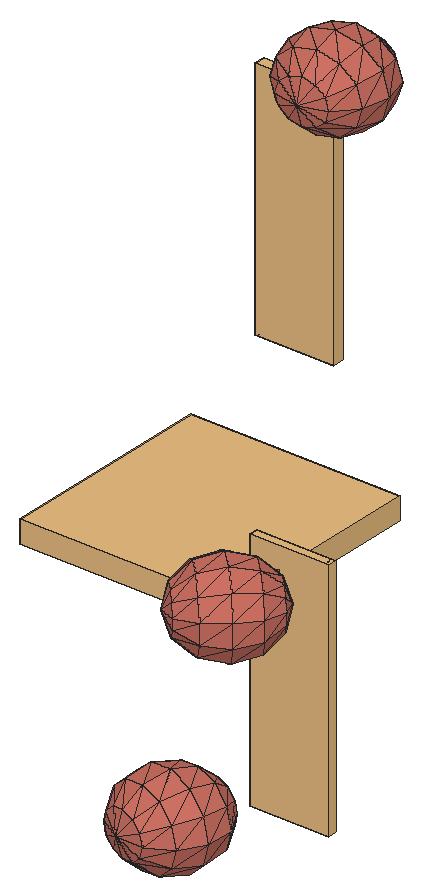
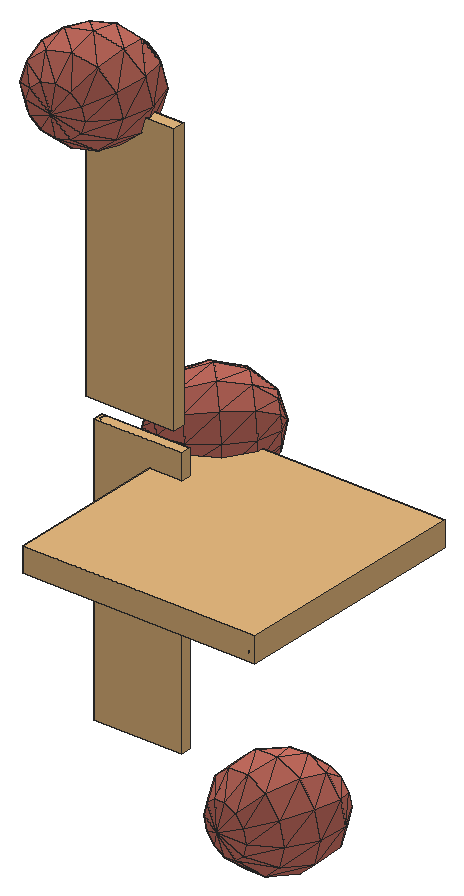
# SketchUp Ruby script. Lengths in inches.
U = 1.inch
M = Sketchup.active_model
def pt(a) = Geom::Point3d.new(a.map { |v| v * U })
def face(e, loops, mat)
  f = e.add_face(loops[0].map { |a| pt(a) })
  loops[1..].each { |l| e.add_face(l.map { |a| pt(a) }).erase! }
  f.material = f.back_material = mat if mat
  f
end
# faces: each face lists its corners as indices into pts; further lists are holes
def faces(e, pts, list, mat = nil) = list.each { |f| face(e, (f[0].is_a?(Array) ? f : [f]).map { |l| l.map { |i| pts[i] } }, mat) }
# xy, xz, yz: faces in a plane at the given z, y or x. An outline is a flat list of corners, or four numbers for a rectangle; further outlines are holes
def ring(l) = l.size == 4 ? [[l[0], l[1]], [l[2], l[1]], [l[2], l[3]], [l[0], l[3]]] : l.each_slice(2).to_a
def flat(e, list, mat, &to3) = list.each { |f| face(e, (f[0].is_a?(Array) ? f : [f]).map { |l| ring(l).map { |u, v| to3.(u, v) } }, mat) }
def xy(e, z, list, mat = nil) = flat(e, list, mat) { |x, y| [x, y, z] }
def xz(e, y, list, mat = nil) = flat(e, list, mat) { |x, z| [x, y, z] }
def yz(e, x, list, mat = nil) = flat(e, list, mat) { |y, z| [x, y, z] }
def lines(e, pts, list) = list.each { |a, b| e.add_line(pt(pts[a]), pt(pts[b])) }
# prism: a flat outline (further loops are holes) pulled along v
def prism(e, loops, v, mat = nil)
  f = face(e, loops, mat); d = Geom::Vector3d.new(v.map { |x| x * U })
  f.pushpull(f.normal.samedirection?(d) ? d.length : -d.length)
end
def box(e, o, s, mat = nil) = prism(e, [[o, [o[0] + s[0], o[1], o[2]], [o[0] + s[0], o[1] + s[1], o[2]], [o[0], o[1] + s[1], o[2]]]], [0, 0, s[2]], mat)
def at(x, y, z, deg = 0) = Geom::Transformation.translation(pt([x, y, z])) * Geom::Transformation.rotation(ORIGIN, Z_AXIS, deg.degrees)
def axes(o, x, y, z) = Geom::Transformation.new([*x, 0, *y, 0, *z, 0, *pt(o).to_a, 1])
def part(name) = M.definitions.add(name)
# library, detail: a bought-in or finely detailed component or shape, given as its bounding box
def library(name, o, s) = part(name).tap { |d| box(d.entities, o, s) }
def detail(e, o, s) = box(e.add_group.entities, o, s)
def put(e, d, t, mat = nil) = e.add_instance(d, t).tap { |i| i.material = mat if mat }
def group(e, t, mat = nil) = e.add_group.tap { |g| g.transformation = t; g.material = mat if mat }.entities
root = M.entities
M.materials.add("green").color = [174, 139, 102]
M.materials.add("vio").color = [206, 114, 100]
c1 = library("3DGeom~125_Defintion",[-500,-52.11,-487.65],[1000,104.22,975.3])
c2 = part("3DGeom~126_Defintion")
p = [[-471.41,-45.23,-481.51],[-492.01,-24.59,-479.28],[-477.71,-31.47,-487.65],[-471.41,-45.23,-481.51],[-477.71,-31.47,-487.65],[-472.84,-38.35,-486.35],
  [-492.01,-24.59,-479.28],[-484.73,-26.43,-485.0625],[-477.71,-31.47,-487.65],[-479.4,-52.11,-467],[-492.01,-24.59,-479.28],[-471.41,-45.23,-481.51],
  [-479.4,-52.11,-467],[-471.41,-45.23,-481.51],[-473.8125,-50.26,-474.43],[-493.7,-45.23,-458.63],[-492.01,-24.59,-479.28],[-479.4,-52.11,-467],
  [-500,-31.47,-464.77],[-492.01,-24.59,-479.28],[-493.7,-45.23,-458.63],[-492.01,-24.59,-479.28],[-497.6,-26.43,-471.85],[-493.7,-45.23,-458.63],
  [-479.4,-52.11,-467],[-486.68,-50.26,-461.22],[-493.7,-45.23,-458.63],[-498.57,-38.35,-459.93],[487.9375,29.11,475.22],[497.875,5.67,462.61],
  [500,13.48,461.23],[487.9375,29.11,475.22],[498.68,21.29,463.39],[487.9375,29.11,475.22],[492.87,-0.05,467.15],[497.875,5.67,462.61],
  [487.9375,29.11,475.22],[498.68,21.29,463.39],[494.26,27.01,468.51],[487.9375,29.11,475.22],[486.33,-2.15,473.66],[492.87,-0.05,467.15],
  [487.9375,29.11,475.22],[480,-0.05,480.37],[486.33,-2.15,473.66],[487.9375,29.11,475.22],[475.59,5.67,485.49],[480,-0.05,480.37],
  [487.9375,29.11,475.22],[474.26,13.48,487.65],[475.59,5.67,485.49],[487.9375,29.11,475.22],[476.39,21.29,486.27],[474.26,13.48,487.65],
  [487.9375,29.11,475.22],[481.39,27.01,481.72],[476.39,21.29,486.27]]
faces(c2.entities,p,[[0,1,2],[3,4,5],[6,7,8],[9,10,11],[12,13,14],[15,16,17],[18,19,20],[21,18,22],
  [23,24,25],[18,26,27],[28,29,30],[31,30,32],[33,34,35],[36,37,38],[39,40,41],[42,43,44],
  [45,46,47],[48,49,50],[51,52,53],[54,55,56]],"green")
c3 = part("3DGeom~196_Defintion")
p = [[141.97,-189.5,-442.47],[-141.24,0,-495.8],[125.58,0,-500],[368.22,-109.41,-337.01],[368.22,-109.41,-337.01],[358.76,0,-370.22],
  [-122.32,218.8125,-429.38],[141.97,189.5,-442.47],[358.76,0,-370.22],[-122.32,-218.81,-429.38],[-370.22,0,-358.76],[-353.83,189.5,-301.23],
  [186.74,-328.22,-285.3125],[394.07,-189.5,-246.27],[394.07,-189.5,-246.27],[368.22,-109.41,-337.01],[358.76,0,-370.22],[368.22,109.41,-337.01],
  [368.22,109.41,-337.01],[186.74,328.22,-285.3125],[-70.62,378.99,-247.9],[-70.62,378.99,-247.9],[186.74,328.22,-285.3125],[-70.62,-378.99,-247.9],
  [-353.83,-189.5,-301.23],[-309.0625,328.22,-144.07],[-309.0625,328.22,-144.07],[-70.62,378.99,-247.9],[368.22,-109.41,-337.01],[358.76,0,-370.22],
  [495.8,0,-141.24],[368.22,109.41,-337.01],[-353.83,-189.5,-301.23],[-500,0,-125.58],[-370.22,0,-358.76],[-370.22,0,-358.76],
  [-490.54,109.41,-92.37],[-370.22,0,-358.76],[-353.83,189.5,-301.23],[394.07,-189.5,-246.27],[394.07,189.5,-246.27],[368.22,109.41,-337.01],
  [186.74,328.22,-285.3125],[394.07,189.5,-246.27],[-309.0625,-328.22,-144.07],[-309.0625,-328.22,-144.07],[-490.54,-109.41,-92.37],[-353.83,-189.5,-301.23],
  [-353.83,-189.5,-301.23],[-353.83,189.5,-301.23],[-464.6875,189.5,-1.63],[-353.83,189.5,-301.23],[-309.0625,328.22,-144.07],[247.9,-378.99,-70.62],
  [-70.62,-378.99,-247.9],[186.74,-328.22,-285.3125],[429.38,-218.8125,-122.32],[247.9,-378.99,-70.62],[186.74,-328.22,-285.3125],[186.74,-328.22,-285.3125],
  [186.74,328.22,-285.3125],[247.9,378.99,-70.62],[186.74,328.22,-285.3125],[-70.62,378.99,-247.9],[0,437.625,0],[186.74,328.22,-285.3125],
  [247.9,378.99,-70.62],[0,-437.625,0],[-309.0625,-328.22,-144.07],[-70.62,-378.99,-247.9],[247.9,-378.99,-70.62],[-70.62,-378.99,-247.9],
  [-309.0625,328.22,-144.07],[-247.9,378.99,70.62],[429.38,218.8125,-122.32],[-247.9,-378.99,70.62],[-309.0625,-328.22,-144.07],[-247.9,-378.99,70.62],
  [-464.6875,-189.5,-1.63],[-309.0625,-328.22,-144.07],[-309.0625,-328.22,-144.07],[-309.0625,328.22,-144.07],[-429.38,218.8125,122.32],[-309.0625,328.22,-144.07],
  [-247.9,378.99,70.62],[464.6875,-189.5,1.63],[490.54,-109.41,92.37],[500,0,125.58],[464.6875,189.5,1.63],[490.54,109.41,92.37],
  [-495.8,0,141.24],[309.0625,328.22,144.07],[309.0625,-328.22,144.07],[247.9,-378.99,-70.62],[309.0625,-328.22,144.07],[247.9,378.99,-70.62],
  [70.62,378.99,247.9],[309.0625,328.22,144.07],[247.9,378.99,-70.62],[70.62,378.99,247.9],[-247.9,-378.99,70.62],[-429.38,-218.8125,122.32],
  [70.62,-378.99,247.9],[309.0625,-328.22,144.07],[-186.74,328.22,285.3125],[-186.74,328.22,285.3125],[70.62,378.99,247.9],[353.83,189.5,301.23],
  [-186.74,-328.22,285.3125],[-247.9,-378.99,70.62],[-186.74,-328.22,285.3125],[-247.9,378.99,70.62],[-394.07,189.5,246.27],[-247.9,378.99,70.62],
  [-394.07,189.5,246.27],[-186.74,328.22,285.3125],[353.83,-189.5,301.23],[370.22,0,358.76],[-186.74,-328.22,285.3125],[-394.07,-189.5,246.27],
  [-394.07,189.5,246.27],[-368.22,-109.41,337.01],[-368.22,-109.41,337.01],[-358.76,0,370.22],[-358.76,0,370.22],[-368.22,109.41,337.01],
  [-368.22,109.41,337.01],[-394.07,189.5,246.27],[353.83,-189.5,301.23],[70.62,-378.99,247.9],[309.0625,-328.22,144.07],[309.0625,328.22,144.07],
  [122.32,218.8125,429.38],[353.83,189.5,301.23],[309.0625,328.22,144.07],[70.62,378.99,247.9],[-141.97,-189.5,442.47],[-394.07,-189.5,246.27],
  [-186.74,-328.22,285.3125],[-368.22,-109.41,337.01],[-394.07,-189.5,246.27],[-186.74,328.22,285.3125],[-394.07,189.5,246.27],[-368.22,109.41,337.01],
  [122.32,-218.8125,429.38],[-186.74,-328.22,285.3125],[70.62,-378.99,247.9],[353.83,-189.5,301.23],[70.62,-378.99,247.9],[-141.97,189.5,442.47],
  [-186.74,-328.22,285.3125],[370.22,0,358.76],[353.83,-189.5,301.23],[353.83,189.5,301.23],[141.24,0,495.8],[353.83,189.5,301.23],
  [370.22,0,358.76],[-125.58,0,500],[-358.76,0,370.22],[370.22,0,358.76]]
faces(c3.entities,p,[[0,1,2],[3,0,2],[4,2,5],[2,1,6],[2,6,7],[8,2,7],[9,10,1],[0,9,1],
  [1,10,11],[1,11,6],[12,9,0],[13,12,0],[14,0,15],[16,7,17],[18,7,19],[7,6,20],
  [7,21,22],[23,24,9],[12,23,9],[9,24,10],[6,11,25],[6,26,27],[28,29,30],[29,31,30],
  [32,33,34],[35,33,36],[37,36,38],[39,28,30],[31,40,30],[41,42,43],[23,44,24],[45,46,47],
  [48,46,33],[49,36,50],[51,50,52],[53,54,55],[56,57,58],[56,59,39],[40,60,61],[62,63,64],
  [65,64,66],[67,68,69],[70,67,71],[63,72,73],[63,73,64],[56,39,30],[40,74,30],[40,61,74],
  [67,75,76],[77,78,79],[80,78,46],[81,50,82],[83,82,84],[85,56,30],[86,85,30],[87,86,30],
  [74,88,30],[88,89,30],[89,87,30],[33,46,90],[36,33,90],[85,57,56],[74,91,88],[74,61,91],
  [46,78,90],[50,36,90],[92,67,93],[85,94,57],[95,96,97],[98,64,99],[100,101,78],[78,101,90],
  [82,50,90],[102,75,67],[103,102,67],[64,73,104],[64,105,106],[86,94,85],[88,107,89],[88,91,107],
  [108,101,109],[102,110,75],[111,82,112],[113,114,115],[86,116,94],[87,116,86],[89,107,117],[89,117,87],
  [118,119,101],[101,119,90],[120,82,90],[87,117,116],[119,121,90],[122,123,90],[124,125,90],[126,127,90],
  [128,129,130],[131,132,133],[134,135,132],[136,137,138],[136,139,140],[141,142,143],[144,145,146],[147,144,148],
  [135,141,149],[135,149,132],[144,136,150],[141,143,149],[151,144,152],[153,132,154],[155,154,156],[157,139,136],
  [157,158,139],[149,143,158],[159,154,144],[149,158,157],[154,136,144],[132,149,157],[132,157,154],[154,157,136]],"vio")
c4 = library("3DGeom~119_Defintion",[-23.33,-500,-162.27],[46.66,1000,324.54])
c5 = part("3DGeom~120_Defintion")
p = [[-7.96,-495.57,-128.3],[7.3,-500,-151.51],[5.77,-494.09,-119.66],[-7.2,-498.52,-144.22],[7.3,-500,-151.51],[-7.96,-495.57,-128.3],
  [7.3,-500,-151.51],[-7.2,-498.52,-144.22],[-0.95,-499.6,-149.76],[5.77,-494.09,-119.66],[7.3,-500,-151.51],[20.27,-495.57,-126.94],
  [7.3,-500,-151.51],[15.35,-499.6,-148.98],[21.03,-498.52,-142.87],[20.27,-495.57,-126.94],[7.3,-500,-151.51],[21.03,-498.52,-142.87],
  [-7.2,-498.52,-144.22],[-7.96,-495.57,-128.3],[-9.76,-497.04,-136.37],[20.27,-495.57,-126.94],[21.03,-498.52,-142.87],[22.83,-497.04,-134.8],
  [-7.96,-495.57,-128.3],[5.77,-494.09,-119.66],[-2.28,-494.49,-122.18],[5.77,-494.09,-119.66],[20.27,-495.57,-126.94],[14.02,-494.49,-121.4],
  [-6.3,500,131.58],[-15.82,491.3,159.83],[-7.77,490.68,162.27],[-6.3,500,131.58],[-7.77,490.68,162.27],[0.48,491.3,160.61],
  [-6.3,500,131.58],[-21.52,493.01,153.92],[-15.82,491.3,159.83],[-6.3,500,131.58],[0.48,491.3,160.61],[6.71,493.01,155.28],
  [-6.3,500,131.58],[-23.33,495.34,146.14],[-21.52,493.01,153.92],[-6.3,500,131.58],[6.71,493.01,155.28],[9.26,495.34,147.71],
  [-6.3,500,131.58],[-20.78,497.67,138.57],[-23.33,495.34,146.14],[-6.3,500,131.58],[9.26,495.34,147.71],[7.45,497.67,139.93],
  [-6.3,500,131.58],[-14.55,499.375,133.24],[-20.78,497.67,138.57],[-6.3,500,131.58],[7.45,497.67,139.93],[1.75,499.375,134.03]]
faces(c5.entities,p,[[0,1,2],[3,4,5],[6,7,8],[9,10,11],[12,13,14],[15,16,17],[18,19,20],[21,22,23],
  [24,25,26],[27,28,29],[30,31,32],[33,34,35],[36,37,38],[39,40,41],[42,43,44],[45,46,47],
  [48,49,50],[51,52,53],[54,55,56],[57,58,59]],"green")
c6 = part("3DGeom~226_Defintion")
p = [[20.8,-212.46,-433.01],[-229.2,0,-445.02],[24.02,0,-500],[268.02,-184,-362.99],[268.02,-184,-362.99],[270.8,0,-421],
  [-231.98,184,-387.01],[20.8,212.47,-433.01],[270.8,0,-421],[-231.98,-184,-387.01],[-421,0,-270.8],[-422.61,106.23,-237.31],
  [-422.61,106.23,-237.31],[12.01,-368,-250],[260.4,-318.7,-204.5],[260.4,-318.7,-204.5],[268.02,-184,-362.99],[270.8,0,-421],
  [268.02,184,-362.99],[-239.6,318.7,-228.52],[268.02,184,-362.99],[12.01,368,-250],[-239.6,318.7,-228.52],[12.01,368,-250],
  [443.41,-106.23,-195.7],[268.02,-184,-362.99],[270.8,0,-421],[445.02,0,-229.2],[268.02,184,-362.99],[-239.6,-318.7,-228.52],
  [-239.6,-318.7,-228.52],[-422.61,-106.23,-237.31],[-231.98,-184,-387.01],[-422.61,-106.23,-237.31],[-231.98,184,-387.01],[-422.61,106.23,-237.31],
  [-427.01,184,-145.8],[-231.98,184,-387.01],[-239.6,318.7,-228.52],[439.02,-184,-104.2],[260.4,-318.7,-204.5],[443.41,106.23,-195.7],
  [260.4,318.7,-204.5],[268.02,184,-362.99],[12.01,368,-250],[260.4,318.7,-204.5],[-421,0,-270.8],[-422.61,-106.23,-237.31],
  [-500,0,-24.02],[-421,0,-270.8],[0,-424.93,0],[-239.6,-318.7,-228.52],[12.01,-368,-250],[250,-368,12.01],
  [12.01,-368,-250],[250,-368,12.01],[12.01,-368,-250],[260.4,-318.7,-204.5],[12.01,368,-250],[-239.6,318.7,-228.52],
  [-250,368,-12.01],[260.4,318.7,-204.5],[0,424.93,0],[-239.6,-318.7,-228.52],[-427.01,-184,-145.8],[-422.61,-106.23,-237.31],
  [-422.61,-106.23,-237.31],[500,0,24.02],[-250,-368,-12.01],[-239.6,-318.7,-228.52],[-250,-368,-12.01],[-239.6,-318.7,-228.52],
  [-239.6,318.7,-228.52],[-433.01,212.47,-20.8],[-239.6,318.7,-228.52],[-250,368,-12.01],[433.01,-212.47,20.8],[250,-368,12.01],
  [439.02,184,-104.2],[250,368,12.01],[260.4,318.7,-204.5],[250,368,12.01],[-250,-368,-12.01],[-433.01,-212.46,-20.8],
  [433.01,212.46,20.8],[-439.02,-184,104.2],[-443.41,-106.23,195.7],[-445.02,0,229.2],[-443.41,106.23,195.7],[-439.02,184,104.2],
  [-260.4,-318.7,204.5],[-250,-368,-12.01],[-260.4,-318.7,204.5],[-250,368,-12.01],[-12.01,-368,250],[-260.4,-318.7,204.5],
  [-250,368,-12.01],[-260.4,318.7,204.5],[-260.4,318.7,204.5],[239.6,-318.7,228.52],[239.6,-318.7,228.52],[250,-368,12.01],
  [-260.4,318.7,204.5],[-12.01,368,250],[250,368,12.01],[-12.01,368,250],[427.01,-184,145.8],[239.6,-318.7,228.52],
  [239.6,318.7,228.52],[250,368,12.01],[-12.01,368,250],[239.6,318.7,228.52],[427.01,184,145.8],[422.61,-106.23,237.31],
  [421,0,270.8],[422.61,106.23,237.31],[-268.01,-184,362.99],[-260.4,-318.7,204.5],[-268.01,-184,362.99],[-260.4,318.7,204.5],
  [231.99,184,387.01],[231.99,184,387.01],[-270.8,0,421],[-268.01,-184,362.99],[-270.8,0,421],[-268.01,184,362.99],
  [-260.4,318.7,204.5],[-268.01,184,362.99],[-20.8,-212.47,433.01],[-260.4,-318.7,204.5],[-12.01,-368,250],[-268.01,-184,362.99],
  [-260.4,-318.7,204.5],[-12.01,368,250],[-260.4,318.7,204.5],[-268.01,184,362.99],[231.99,-184,387.01],[-12.01,-368,250],
  [239.6,-318.7,228.52],[231.99,-184,387.01],[239.6,318.7,228.52],[-20.8,212.47,433.01],[231.99,184,387.01],[239.6,318.7,228.52],
  [-268.01,184,362.99],[-270.8,0,421],[421,0,270.8],[231.99,-184,387.01],[422.61,-106.23,237.31],[422.61,106.23,237.31],
  [229.2,0,445.02],[422.61,106.23,237.31],[421,0,270.8],[231.99,-184,387.01],[-12.01,-368,250],[421,0,270.8],
  [231.99,-184,387.01],[-24.02,0,500],[-270.8,0,421],[231.99,-184,387.01]]
faces(c6.entities,p,[[0,1,2],[3,0,2],[4,2,5],[2,1,6],[2,6,7],[8,2,7],[0,9,1],[9,10,1],
  [1,10,11],[1,12,6],[13,9,0],[14,13,0],[15,0,16],[17,7,18],[7,6,19],[20,7,21],
  [7,22,23],[24,25,26],[24,26,27],[27,26,28],[13,29,9],[30,31,32],[9,33,10],[34,35,36],
  [37,36,38],[39,40,25],[39,25,24],[27,28,41],[41,28,42],[43,44,45],[46,47,48],[35,49,48],
  [50,51,52],[53,50,54],[55,56,57],[58,59,60],[61,58,62],[58,60,62],[63,64,65],[66,64,48],
  [36,35,48],[24,27,67],[27,41,67],[50,68,69],[70,64,71],[72,36,73],[74,73,75],[76,77,40],
  [76,40,39],[41,42,78],[78,42,79],[80,62,81],[39,24,67],[41,78,67],[82,83,64],[64,83,48],
  [73,36,48],[76,39,67],[78,84,67],[78,79,84],[83,85,48],[85,86,48],[86,87,48],[87,88,48],
  [88,89,48],[89,73,48],[90,83,91],[92,85,83],[93,73,89],[94,68,50],[94,95,68],[96,89,97],
  [62,60,98],[99,94,50],[100,50,101],[62,102,103],[104,62,105],[106,107,77],[106,77,76],[84,79,108],
  [109,110,111],[106,76,67],[84,112,67],[84,108,112],[113,106,67],[114,113,67],[115,114,67],[112,115,67],
  [116,85,117],[118,86,85],[119,89,88],[113,107,106],[112,120,115],[112,108,121],[122,86,123],[124,87,86],
  [125,88,87],[126,88,127],[128,129,130],[128,131,132],[133,134,135],[136,137,138],[113,139,107],[140,141,142],
  [143,133,141],[144,87,145],[146,147,148],[149,142,150],[151,150,152],[153,128,154],[133,135,141],[155,150,156],
  [157,131,128],[157,158,131],[141,135,158],[150,128,159],[142,141,157],[142,157,150],[141,158,157],[150,157,128]],"vio")
c7 = part("3DGeom~229_Defintion")
p = [[135.68,-61.63,-498.07],[-132.16,91.58,-492.59],[133.7,52.87,-500],[363.74,0,-373.43],[180.3,153.22,-454.61],[-51.45,265.375,-413.98],
  [185.71,-159.63,-449.34],[-128.73,-106.76,-489.25],[-362.61,105.75,-353.2],[-269.41,306.43,-262.42],[-269.41,306.43,-262.42],[-42.08,-276.49,-404.84],
  [-358.65,-123.27,-349.34],[262.99,212.5,-374.0625],[91.78,368.07,-274.47],[91.78,368.07,-274.47],[270.39,-214.85,-366.86],[-51.45,265.375,-413.98],
  [-269.41,306.43,-262.42],[-104.02,425.01,-101.32],[-51.45,265.375,-413.98],[91.78,368.07,-274.47],[104.59,-372.13,-261.99],[-258.59,-319.26,-251.875],
  [-42.08,-276.49,-404.84],[104.59,-372.13,-261.99],[-258.59,-319.26,-251.875],[359.62,214.85,-279.94],[262.99,212.5,-374.0625],[259.15,372.13,-111.44],
  [262.99,212.5,-374.0625],[259.15,372.13,-111.44],[359.62,214.85,-279.94],[367.02,-212.5,-272.74],[449.71,-153.21,-192.19],[367.02,-212.5,-272.74],
  [363.74,0,-373.43],[496.3125,-52.87,-146.8],[363.74,0,-373.43],[494.33,61.64,-148.73],[363.74,0,-373.43],[359.62,214.85,-279.94],
  [444.3,159.63,-197.46],[363.74,0,-373.43],[363.74,0,-373.43],[367.02,-212.5,-272.74],[104.59,-372.13,-261.99],[270.39,-214.85,-366.86],
  [-358.65,-123.27,-349.34],[-495.9,91.58,-119.16],[-362.61,105.75,-353.2],[-362.61,105.75,-353.2],[-415.1875,265.38,-40.55],[-362.61,105.75,-353.2],
  [-415.1875,265.38,-40.55],[-269.41,306.43,-262.42],[-258.59,-319.26,-251.875],[-492.47,-106.76,-115.82],[-358.65,-123.27,-349.34],[-358.65,-123.27,-349.34],
  [405.8125,276.49,31.41],[259.15,372.13,-111.44],[89.24,429.7,86.92],[259.15,372.13,-111.44],[367.02,-212.5,-272.74],[271.96,-368.07,-98.97],
  [104.59,-372.13,-261.99],[271.96,-368.07,-98.97],[367.02,-212.5,-272.74],[-415.1875,265.38,-40.55],[-271.96,368.07,98.97],[104.59,-372.13,-261.99],
  [-89.24,-429.7,-86.92],[-258.59,-319.26,-251.875],[104.59,-372.13,-261.99],[-405.8125,-276.49,-31.41],[-258.59,-319.26,-251.875],[-258.59,-319.26,-251.875],
  [-405.8125,-276.49,-31.41],[492.47,106.75,115.82],[415.1875,-265.375,40.55],[271.96,-368.07,-98.97],[495.9,-91.58,119.16],[-496.3125,52.87,146.8],
  [-449.71,153.21,192.19],[-415.1875,265.38,-40.55],[-494.33,-61.64,148.73],[259.15,372.13,-111.44],[258.59,319.26,251.875],[405.8125,276.49,31.41],
  [259.15,372.13,-111.44],[258.59,319.26,251.875],[-104.59,372.13,261.99],[104.02,-425.01,101.32],[415.1875,-265.375,40.55],[-259.15,-372.13,111.44],
  [-405.8125,-276.49,-31.41],[-415.1875,265.38,-40.55],[-367.02,212.5,272.74],[-415.1875,265.38,-40.55],[-367.02,212.5,272.74],[-271.96,368.07,98.97],
  [-259.15,-372.13,111.44],[-444.3,-159.63,197.46],[358.65,123.27,349.34],[258.59,319.26,251.875],[415.1875,-265.375,40.55],[269.41,-306.43,262.42],
  [269.41,-306.43,262.42],[42.08,276.49,404.84],[42.08,276.49,404.84],[258.59,319.26,251.875],[-367.02,212.5,272.74],[-270.39,214.85,366.86],
  [-270.39,214.85,366.86],[-91.78,-368.07,274.47],[-259.15,-372.13,111.44],[-359.62,-214.85,279.94],[-359.62,-214.85,279.94],[362.61,-105.75,353.2],
  [269.41,-306.43,262.42],[-363.74,0,373.43],[-367.02,212.5,272.74],[258.59,319.26,251.875],[42.08,276.49,404.84],[128.73,106.76,489.25],
  [258.59,319.26,251.875],[358.65,123.27,349.34],[-104.59,372.13,261.99],[-270.39,214.85,366.86],[-185.71,159.63,449.34],[-104.59,372.13,261.99],
  [51.45,-265.375,413.98],[362.61,-105.75,353.2],[51.45,-265.375,413.98],[269.41,-306.43,262.42],[-367.02,212.5,272.74],[-363.74,0,373.43],
  [-262.99,-212.5,374.0625],[-359.62,-214.85,279.94],[51.45,-265.375,413.98],[-262.99,-212.5,374.0625],[-91.78,-368.07,274.47],[-359.62,-214.85,279.94],
  [-262.99,-212.5,374.0625],[-363.74,0,373.43],[358.65,123.27,349.34],[132.16,-91.58,492.59],[362.61,-105.75,353.2],[358.65,123.27,349.34],
  [362.61,-105.75,353.2],[51.45,-265.375,413.98],[-363.74,0,373.43],[-262.99,-212.5,374.0625],[-180.3,-153.22,454.61],[-363.74,0,373.43],
  [-133.7,-52.87,500],[-363.74,0,373.43],[-135.68,61.63,498.07],[-363.74,0,373.43],[-363.74,0,373.43],[51.45,-265.375,413.98],
  [-262.99,-212.5,374.0625],[51.45,-265.375,413.98]]
faces(c7.entities,p,[[0,1,2],[0,2,3],[2,4,3],[2,1,5],[2,5,4],[6,7,0],[6,0,3],[0,7,1],
  [7,8,1],[1,8,9],[1,10,5],[11,12,7],[6,11,7],[7,12,8],[4,13,3],[4,5,14],
  [4,15,13],[16,11,6],[16,6,3],[17,18,19],[20,19,21],[22,23,24],[16,25,11],[11,26,12],
  [13,27,3],[28,21,29],[30,31,32],[33,16,3],[34,35,36],[37,34,38],[39,37,40],[41,42,43],
  [42,39,44],[45,46,47],[48,49,50],[51,49,52],[53,54,55],[56,57,58],[59,57,49],[41,60,42],
  [41,61,60],[21,19,62],[21,62,63],[64,65,66],[34,67,68],[18,69,70],[18,70,19],[71,72,73],
  [65,72,74],[72,75,76],[77,78,57],[42,79,39],[42,60,79],[34,80,81],[37,80,34],[39,79,82],
  [39,82,37],[37,82,80],[57,83,49],[49,83,84],[49,84,85],[78,86,57],[57,86,83],[87,88,89],
  [90,62,91],[19,70,92],[19,92,62],[65,93,72],[94,93,65],[72,95,96],[93,95,72],[97,84,98],
  [99,100,101],[102,103,78],[78,103,86],[60,104,79],[60,105,104],[106,107,93],[82,108,80],[62,92,109],
  [62,110,111],[70,112,113],[70,114,92],[93,115,95],[107,115,93],[116,117,103],[115,118,95],[79,104,119],
  [79,119,82],[82,119,120],[83,86,121],[84,83,121],[86,103,121],[122,84,121],[103,117,121],[123,124,125],
  [126,125,127],[128,129,130],[131,130,124],[107,132,115],[133,134,135],[129,136,137],[115,138,139],[140,141,142],
  [143,144,145],[146,147,148],[149,125,147],[150,147,151],[130,129,152],[153,154,155],[154,156,157],[156,158,159],
  [158,130,160],[161,154,162],[124,130,158],[124,158,125],[147,154,163],[147,156,154],[125,156,147],[125,158,156]],"vio")
c8 = library("3DGeom~7_Defintion",[-18.22,-500,-162.45],[36.44,1000,324.9])
c9 = part("3DGeom~8_Defintion")
p = [[-16.01,-498.52,-143.51],[-1.98,-500,-151.67],[-15.8,-495.57,-127.57],[-1.98,-500,-151.67],[-16.01,-498.52,-143.51],[-10.11,-499.6,-149.43],
  [-15.8,-495.57,-127.57],[-1.98,-500,-151.67],[-1.57,-494.09,-119.79],[-1.98,-500,-151.67],[6.21,-499.6,-149.64],[12.25,-498.52,-143.88],
  [12.46,-495.57,-127.94],[12.25,-498.52,-143.88],[12.46,-495.57,-127.94],[12.25,-498.52,-143.88],[14.54,-497.04,-135.94],[-16.01,-498.52,-143.51],
  [-15.8,-495.57,-127.57],[-18.09,-497.04,-135.52],[-1.57,-494.09,-119.79],[12.46,-495.57,-127.94],[6.57,-494.49,-122.03],[-15.8,-495.57,-127.57],
  [-1.57,-494.09,-119.79],[-9.75,-494.49,-121.82],[1.71,500,131.72],[-6.08,491.3,160.5],[2.11,490.68,162.45],[1.71,500,131.72],
  [2.11,490.68,162.45],[10.24,491.3,160.28],[1.71,500,131.72],[-12.12,493.01,154.95],[-6.08,491.3,160.5],[1.71,500,131.72],
  [10.24,491.3,160.28],[16.14,493.01,154.58],[1.71,500,131.72],[-14.41,495.34,147.3],[-12.12,493.01,154.95],[1.71,500,131.72],
  [16.14,493.01,154.58],[18.22,495.34,146.87],[1.71,500,131.72],[-12.32,497.67,139.58],[-14.41,495.34,147.3],[1.71,500,131.72],
  [18.22,495.34,146.87],[15.9375,497.67,139.22],[1.71,500,131.72],[-6.42,499.375,133.88],[-12.32,497.67,139.58],[1.71,500,131.72],
  [15.9375,497.67,139.22],[9.89,499.375,133.67]]
faces(c9.entities,p,[[0,1,2],[3,4,5],[6,7,8],[9,10,11],[12,7,13],[8,7,12],[14,15,16],[17,18,19],
  [20,21,22],[23,24,25],[26,27,28],[29,30,31],[32,33,34],[35,36,37],[38,39,40],[41,42,43],
  [44,45,46],[47,48,49],[50,51,52],[53,54,55]],"green")
g1 = group(root,at(15.3125,134.49,26.21))
put(g1,c1,axes([2.03,0.28,10.94],[0,0.0008,0],[0,0,-0.0008],[-0.0008,0,0]),"green")
put(g1,c2,axes([2.03,0.28,10.94],[0,0.0008,0],[0,0,-0.0008],[-0.0008,0,0]),"green")
g2 = group(root,at(15.3125,134.49,26.21))
put(g2,c3,axes([2.05,0.07,10.04],[0,0.00038,0],[0,0,-0.00038],[-0.00038,0,0]),"vio")
g3 = group(root,at(15.3125,134.49,26.21))
put(g3,c4,axes([2.14,0.56,11.89],[0,0.00091,0],[0,0,-0.00091],[-0.00091,0,0]),"green")
put(g3,c5,axes([2.14,0.56,11.89],[0,0.00091,0],[0,0,-0.00091],[-0.00091,0,0]),"green")
g4 = group(root,at(15.3125,134.49,26.21))
put(g4,c6,axes([2.27,0.57,12.375],[0,0.00039,0],[0,0,-0.00039],[-0.00039,0,0]),"vio")
g5 = group(root,at(15.3125,134.49,26.21))
put(g5,c7,axes([2.4375,-0.15,10.98],[0,0.00037,0],[0,0,-0.00037],[-0.00037,0,0]),"vio")
g6 = group(root,at(15.3125,134.49,26.21))
put(g6,c8,axes([2.46,0.13,10.61],[0,0.00091,0],[0,0,-0.00091],[-0.00091,0,0]),"green")
put(g6,c9,axes([2.46,0.13,10.61],[0,0.00091,0],[0,0,-0.00091],[-0.00091,0,0]),"green")
